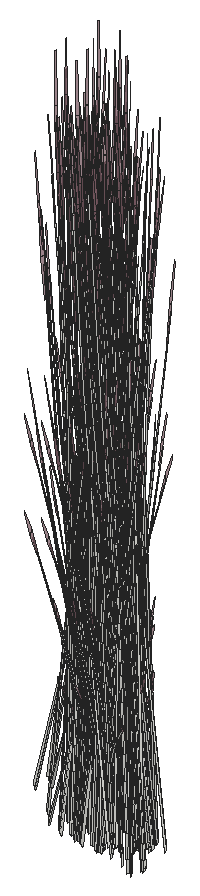
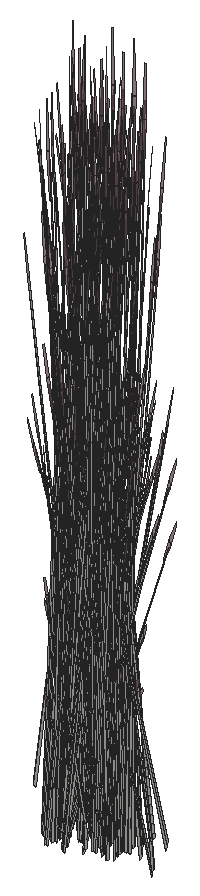
# SketchUp Ruby script. Lengths in inches.
U = 1.inch
M = Sketchup.active_model
def pt(a) = Geom::Point3d.new(a.map { |v| v * U })
def face(e, loops, mat)
  f = e.add_face(loops[0].map { |a| pt(a) })
  loops[1..].each { |l| e.add_face(l.map { |a| pt(a) }).erase! }
  f.material = f.back_material = mat if mat
  f
end
# faces: each face lists its corners as indices into pts; further lists are holes
def faces(e, pts, list, mat = nil) = list.each { |f| face(e, (f[0].is_a?(Array) ? f : [f]).map { |l| l.map { |i| pts[i] } }, mat) }
# xy, xz, yz: faces in a plane at the given z, y or x. An outline is a flat list of corners, or four numbers for a rectangle; further outlines are holes
def ring(l) = l.size == 4 ? [[l[0], l[1]], [l[2], l[1]], [l[2], l[3]], [l[0], l[3]]] : l.each_slice(2).to_a
def flat(e, list, mat, &to3) = list.each { |f| face(e, (f[0].is_a?(Array) ? f : [f]).map { |l| ring(l).map { |u, v| to3.(u, v) } }, mat) }
def xy(e, z, list, mat = nil) = flat(e, list, mat) { |x, y| [x, y, z] }
def xz(e, y, list, mat = nil) = flat(e, list, mat) { |x, z| [x, y, z] }
def yz(e, x, list, mat = nil) = flat(e, list, mat) { |y, z| [x, y, z] }
def lines(e, pts, list) = list.each { |a, b| e.add_line(pt(pts[a]), pt(pts[b])) }
# prism: a flat outline (further loops are holes) pulled along v
def prism(e, loops, v, mat = nil)
  f = face(e, loops, mat); d = Geom::Vector3d.new(v.map { |x| x * U })
  f.pushpull(f.normal.samedirection?(d) ? d.length : -d.length)
end
def box(e, o, s, mat = nil) = prism(e, [[o, [o[0] + s[0], o[1], o[2]], [o[0] + s[0], o[1] + s[1], o[2]], [o[0], o[1] + s[1], o[2]]]], [0, 0, s[2]], mat)
def at(x, y, z, deg = 0) = Geom::Transformation.translation(pt([x, y, z])) * Geom::Transformation.rotation(ORIGIN, Z_AXIS, deg.degrees)
def axes(o, x, y, z) = Geom::Transformation.new([*x, 0, *y, 0, *z, 0, *pt(o).to_a, 1])
def part(name) = M.definitions.add(name)
# library, detail: a bought-in or finely detailed component or shape, given as its bounding box
def library(name, o, s) = part(name).tap { |d| box(d.entities, o, s) }
def detail(e, o, s) = box(e.add_group.entities, o, s)
def put(e, d, t, mat = nil) = e.add_instance(d, t).tap { |i| i.material = mat if mat }
def group(e, t, mat = nil) = e.add_group.tap { |g| g.transformation = t; g.material = mat if mat }.entities
root = M.entities
M.materials.add("LightPink_Translucent").color = [144, 107, 117]
M.materials["LightPink_Translucent"].alpha = 0.75
c1 = part("blade")
p = [[2.15,0.21,22],[0,0.17,0],[0.09,0.45,0],[2.18,0.31,22],[2.29,0.31,22],[0.38,0.45,0],
  [2.48,0.24,33],[2.49,0.24,33],[2.48,0.22,33]]
faces(c1.entities,p,[[0,1,2,3],[4,5,2,3],[6,3,4,7],[8,0,3,6]])
c2 = part("seeds")
p = [[0.3,-0.1,1.38],[-0.01,-0.03,1.59],[-0.01,-0.03,0.03],[0.14,-0.07,-0.07],[0.29,-0.03,3],[0.15,0.01,3.11]]
faces(c2.entities,p,[[0,1,2,3],[1,0,4,5]],"LightPink_Translucent")
c3 = part("blade with seeds")
put(c3.entities,c1,at(0,0,0))
put(c3.entities,c2,axes([2.4,0.25,30.99],[1.5799,-0.05474,1.17369],[-0.12525,1.92788,0.29478],[-0.07173,-0.02425,1.56792]))
put(root,c3,axes([350.7,355.2,622.53],[0.29332,0.1301,-0.35414],[-0.08555,0.37955,0.4572],[0.11809,-0.0348,0.87481]))
put(root,c3,axes([354.22,355.91,620.47],[0.10196,-0.46348,0.17642],[0.3731,0.13116,0.35086],[-0.06445,0.00226,1.60407]))
put(root,c3,axes([353.96,354.95,620.3],[-0.32829,-0.4014,-0.06131],[0.32849,-0.40164,0],[-0.01146,-0.01402,1.75571]))
put(root,c3,axes([356.95,354.6,621.875],[0.14639,-0.01056,1.71376],[-0.09712,0.45778,0.13857],[-0.20862,-0.02831,0.73262]))
put(root,c3,axes([350.85,355.125,619.98],[-0.22732,0.05597,1.41583],[-0.03618,-0.44548,0.08104],[0.15921,-0.06743,0.80566]))
put(root,c3,axes([351.1,354.83,619.49],[-0.01845,-0.0708,1.76342],[0.12793,-0.41416,-0.26939],[0.12905,-0.00596,0.30037]))
put(root,c3,axes([355.63,354.99,620.67],[-0.35635,0.30962,-0.29095],[-0.23697,-0.43749,-0.50002],[-0.08792,-0.04443,1.59708]))
put(root,c3,axes([349.9,354.73,621.875],[-0.14639,0.01056,1.71376],[0.09712,-0.45778,0.13857],[0.20862,0.02831,0.73262]))
put(root,c3,axes([353.3,354.49,620.36],[0.15345,0.52148,0.45755],[-0.43845,0.18134,0.17955],[0.00536,-0.09582,1.58856]))
put(root,c3,axes([353.66,355.78,620.2],[-0.11516,-0.40207,0],[0.32884,-0.1408,0],[0,0,1.54371]))
put(root,c3,axes([354.83,355.64,620.03],[-0.08291,-0.40636,-0.30978],[0.32928,-0.11539,0.30978],[-0.06638,-0.04686,1.38974]))
put(root,c3,axes([350.44,355.16,622.98],[0.31014,-0.20596,-0.71045],[0.17284,0.42397,0.08574],[0.14985,-0.04816,1.00501]))
put(root,c3,axes([351.48,354.71,622.72],[0.04898,-0.07104,1.74944],[-0.06269,-0.43574,-0.27667],[0.12289,-0.08262,0.14031]))
put(root,c3,axes([354.81,354.73,620.47],[-0.2773,-0.3397,0.17642],[0.27945,-0.32949,0.35086],[-0.03063,0.06937,1.60407]))
put(root,c3,axes([356.03,355.13,620.46],[-0.34464,-0.37536,-0.25192],[0.29,-0.42149,0.5513],[-0.0928,0.04391,1.68216]))
put(root,c3,axes([355.41,354.77,620.21],[-0.21202,-0.39143,-0.44739],[0.32115,-0.27564,0.21531],[-0.06861,-0.04843,1.43643]))
put(root,c3,axes([353.85,354.53,620.21],[0,-0.53961,0],[0.44133,0,0],[0,0,1.79456]))
put(root,c3,axes([353.4375,354.63,620.43],[0.39767,0.22603,0.24065],[-0.19139,0.46966,0.50002],[0,-0.10827,1.60543]))
put(root,c3,axes([354.07,354.75,620.29],[0,0.53934,-0.05637],[-0.44133,0,0],[0,0.01695,1.79368]))
put(root,c3,axes([353.31,354.32,620.72],[-0.38326,0.02879,0.44739],[-0.03466,-0.47788,-0.21531],[0.06861,-0.04843,1.43643]))
put(root,c3,axes([355.86,355.05,620.21],[-0.38326,0.02879,-0.44739],[-0.03466,-0.47788,0.21531],[-0.06861,0.04843,1.43643]))
put(root,c3,axes([353.13,353.5,620.47],[-0.10196,0.46348,0.17642],[-0.3731,-0.13116,0.35086],[0.06445,-0.00226,1.60407]))
put(root,c3,axes([357.39,354.17,622.98],[-0.35281,-0.01123,-0.71045],[0.0237,-0.47284,0.08574],[-0.14947,-0.0499,1.00501]))
put(root,c3,axes([355.13,355.85,620.48],[0.33032,0.23318,0.49651],[-0.19744,0.41812,0],[-0.07523,-0.05311,1.57504]))
put(root,c3,axes([357.1,354.28,620.59],[0.06891,0.12984,1.43002],[-0.15879,0.35293,-0.30754],[-0.16304,-0.08436,0.61141]))
put(root,c3,axes([355.4375,354.99,620.4375],[0.09355,-0.55261,-0.23429],[0.44354,0.09633,0.51271],[-0.0775,-0.07631,1.5644]))
put(root,c3,axes([356.82,354.99,622.53],[-0.29332,-0.1301,-0.35414],[0.08555,-0.37955,0.4572],[-0.11809,0.0348,0.87481]))
put(root,c3,axes([354.26,353.52,620.47],[-0.37926,0.12378,0.17642],[-0.09365,-0.46065,0.35086],[0.03382,0.06712,1.60407]))
put(root,c3,axes([355.6,355.125,620.62],[-0.06809,0.4162,0.1448],[-0.33266,-0.07225,-0.41347],[-0.06054,-0.04274,1.26744]))
put(root,c3,axes([354.48,354.39,620.48],[0,0.46636,0.49651],[-0.39487,0,0],[0,-0.10622,1.57504]))
put(root,c3,axes([353.64,354.19,620.36],[-0.29264,0.42323,0.45755],[-0.34767,-0.3736,0.17955],[0.07055,-0.04224,1.58856]))
put(root,c3,axes([354.14,354.86,620.21],[0.24637,0.30123,0],[-0.24637,0.30123,0],[0,0,1.69266]))
put(root,c3,axes([354.13,354.51,620.72],[0.17124,-0.42022,0.44739],[0.35581,0.20224,-0.21531],[0,0.09687,1.43643]))
put(root,c3,axes([357.27,354.27,622.68],[-0.25628,0.30892,-0.51099],[-0.22444,-0.32634,-0.3958],[-0.13021,-0.047,0.97773]))
put(root,c3,axes([356.86,355.16,619.49],[0.00895,0.0735,1.76342],[-0.18044,0.38382,-0.26939],[-0.12817,-0.01935,0.30037]))
put(root,c3,axes([354.02,354.41,620.38],[-0.44609,-0.09826,0.49198],[0.09078,-0.55493,0.19306],[0.06519,0.05359,1.70813]))
put(root,c3,axes([356.91,353.4,622.71],[0.02617,0.04654,1.77383],[-0.12614,0.41836,-0.16761],[-0.12775,0.00303,0.31391]))
put(root,c3,axes([354.15,354.66,620.21],[0.39487,0,0],[0,0.48281,0],[0,0,1.78407]))
put(root,c3,axes([356.89,354.94,622.73],[0.09971,-0.42522,0.48003],[0.32782,0.1454,0.3958],[-0.12892,0.02555,0.9933]))
put(root,c3,axes([353.77,354.12,620.72],[-0.21202,-0.39143,0.44739],[0.32115,-0.27564,-0.21531],[0.06861,0.04843,1.43643]))
put(root,c3,axes([357.41,353.94,623.03],[-0.0189,0.47427,-0.1216],[-0.35781,-0.01296,-0.67495],[-0.13781,-0.03295,1.02557]))
put(root,c3,axes([357.18,353.97,622.53],[-0.20082,-0.29199,-0.35414],[0.2293,-0.2764,0.4572],[-0.1165,-0.04206,0.87481]))
put(root,c3,axes([356.86,354.83,622.73],[-0.12963,-0.31798,0.0643],[0.23638,-0.15564,0.50621],[-0.1042,0.03071,0.77189]))
put(root,c3,axes([358.49,354.61,621.875],[0.14639,-0.01056,1.71376],[-0.09712,0.45778,0.13857],[-0.20862,-0.02831,0.73262]))
put(root,c3,axes([355.49,354.73,620.36],[0.44609,0.09826,0.45755],[-0.09078,0.55493,0.17955],[-0.06519,-0.05359,1.58856]))
put(root,c3,axes([356.69,354.67,620.77],[0.22533,-0.03337,1.1486],[-0.14293,0.29403,0.84392],[-0.11135,-0.04411,0.25299]))
put(root,c3,axes([355.375,354.63,620.72],[-0.17124,0.42022,0.44739],[-0.35581,-0.20224,-0.21531],[0,-0.09687,1.43643]))
put(root,c3,axes([353.91,354.01,620.62],[0.06809,-0.4162,0.1448],[0.33266,0.07225,-0.41347],[0.06054,0.04274,1.26744]))
put(root,c3,axes([355.25,355.61,620.47],[0.37926,-0.12378,0.17642],[0.09365,0.46065,0.35086],[-0.03382,-0.06712,1.60407]))
put(root,c3,axes([355.74,355.6875,620.2],[-0.35581,-0.20937,0],[0.17124,-0.43505,0],[0,0,1.62707]))
put(root,c3,axes([354.38,353.29,620.48],[-0.33032,-0.23318,0.49651],[0.19744,-0.41812,0],[0.07523,0.05311,1.57504]))
put(root,c3,axes([354.09,355.72,620.18],[0.37054,-0.15823,-0.19198],[0.1302,0.45581,0.00008],[0.0409,-0.01749,1.73897]))
put(root,c3,axes([357.13,354.95,623.05],[0.29332,0.1301,0.35414],[-0.08555,0.37955,-0.4572],[-0.11809,0.0348,0.87481]))
put(root,c3,axes([356.38,355.64,620.47],[0.10196,-0.46348,0.17642],[0.3731,0.13116,0.35086],[-0.06445,0.00226,1.60407]))
put(root,c3,axes([357.28,353.86,622.73],[0.01777,-0.35463,0.0643],[0.26836,0.00972,0.50621],[-0.1028,-0.03711,0.77189]))
put(root,c3,axes([356.11,354.68,620.3],[-0.32829,-0.4014,-0.06131],[0.32849,-0.40164,0],[-0.01146,-0.01402,1.75571]))
put(root,c3,axes([356.2,354.82,620.72],[0.38326,-0.02879,0.44739],[0.03466,0.47788,-0.21531],[-0.06861,0.04843,1.43643]))
put(root,c3,axes([358.04,355.82,620.06],[-0.36714,-0.07646,-0.62353],[0.07747,-0.47163,-0.16365],[-0.10956,-0.05715,1.37633]))
put(root,c3,axes([354.1,354.37,620.21],[0.21202,0.39143,-0.44739],[-0.32115,0.27564,0.21531],[0.06861,0.04843,1.43643]))
put(root,c3,axes([357.46,354.13,623.05],[0.20082,0.29199,0.35414],[-0.2293,0.2764,-0.4572],[-0.1165,-0.04206,0.87481]))
put(root,c3,axes([355.45,354.22,620.36],[0.15345,0.52148,0.45755],[-0.43845,0.18134,0.17955],[0.00536,-0.09582,1.58856]))
put(root,c3,axes([358.92,354.18,622.98],[-0.35281,-0.01123,-0.71045],[0.0237,-0.47284,0.08574],[-0.14947,-0.0499,1.00501]))
put(root,c3,axes([355.82,355.51,620.2],[-0.11516,-0.40207,0],[0.32884,-0.1408,0],[0,0,1.54371]))
put(root,c3,axes([358.64,354.3,620.59],[0.06891,0.12984,1.43002],[-0.15879,0.35293,-0.30754],[-0.16304,-0.08436,0.61141]))
put(root,c3,axes([357.56,356.71,620.02],[-0.33032,-0.23318,-0.49651],[0.19744,-0.41812,0],[-0.07523,-0.05311,1.57504]))
put(root,c3,axes([359.07,351.34,621.875],[0.12246,-0.09864,1.71376],[0.1031,0.45582,0.13857],[-0.19225,0.10302,0.73262]))
put(root,c3,axes([358.36,355,622.53],[-0.29332,-0.1301,-0.35414],[0.08555,-0.37955,0.4572],[-0.11809,0.0348,0.87481]))
put(root,c3,axes([358.6875,352.12,620.59],[0.12266,0.03828,1.43002],[0.07906,0.39104,-0.30754],[-0.16661,0.0732,0.61141]))
put(root,c3,axes([354.68,353.5,620.03],[0.08291,0.40636,-0.30978],[-0.32928,0.11539,0.30978],[0.06638,0.04686,1.38974]))
put(root,c3,axes([353.875,354.15,620.67],[0.35635,-0.30962,-0.29095],[0.23697,0.43749,-0.50002],[0.08792,0.04443,1.59708]))
put(root,c3,axes([358.81,354.28,622.68],[-0.25628,0.30892,-0.51099],[-0.22444,-0.32634,-0.3958],[-0.13021,-0.047,0.97773]))
put(root,c3,axes([358.39,355.17,619.49],[0.00895,0.0735,1.76342],[-0.18044,0.38382,-0.26939],[-0.12817,-0.01935,0.30037]))
put(root,c3,axes([356.96,354.46,620.47],[-0.2773,-0.3397,0.17642],[0.27945,-0.32949,0.35086],[-0.03063,0.06937,1.60407]))
put(root,c3,axes([356,354.26,620.21],[0,-0.53961,0],[0.44133,0,0],[0,0,1.79456]))
put(root,c3,axes([357.2,353.48,620.13],[-0.10181,0.3808,-0.03893],[-0.31336,-0.11714,-0.17649],[-0.04758,-0.06228,0.58215]))
put(root,c3,axes([355.59,354.36,620.43],[0.39767,0.22603,0.24065],[-0.19139,0.46966,0.50002],[0,-0.10827,1.60543]))
put(root,c3,axes([356.23,354.48,620.29],[0,0.53934,-0.05637],[-0.44133,0,0],[0,0.01695,1.79368]))
put(root,c3,axes([358.44,353.41,622.71],[0.02617,0.04654,1.77383],[-0.12614,0.41836,-0.16761],[-0.12775,0.00303,0.31391]))
put(root,c3,axes([355.47,354.04,620.72],[-0.38326,0.02879,0.44739],[-0.03466,-0.47788,-0.21531],[0.06861,-0.04843,1.43643]))
put(root,c3,axes([355.29,353.22,620.47],[-0.10196,0.46348,0.17642],[-0.3731,-0.13116,0.35086],[0.06445,-0.00226,1.60407]))
put(root,c3,axes([358.45,355.89,620.67],[-0.35635,0.30962,-0.29095],[-0.23697,-0.43749,-0.50002],[-0.08792,-0.04443,1.59708]))
put(root,c3,axes([358.43,354.95,622.73],[0.09971,-0.42522,0.48003],[0.32782,0.1454,0.3958],[-0.12892,0.02555,0.9933]))
put(root,c3,axes([352.98,353.87,619.59],[-0.3474,0.18671,1.28929],[-0.11057,-0.53572,0.50096],[0.21332,0.00891,1.46642]))
put(root,c3,axes([358.94,353.95,623.03],[-0.0189,0.47427,-0.1216],[-0.35781,-0.01296,-0.67495],[-0.13781,-0.03295,1.02557]))
put(root,c3,axes([358.71,353.99,622.53],[-0.20082,-0.29199,-0.35414],[0.2293,-0.2764,0.4572],[-0.1165,-0.04206,0.87481]))
put(root,c3,axes([358.4,354.84,622.73],[-0.12963,-0.31798,0.0643],[0.23638,-0.15564,0.50621],[-0.1042,0.03071,0.77189]))
put(root,c3,axes([357.03,355.22,620.375],[-0.44133,0,0],[0,-0.52122,-0.51607],[0,-0.11871,1.63711]))
put(root,c3,axes([357.65,356.54,620.03],[-0.08291,-0.40636,-0.30978],[0.32928,-0.11539,0.30978],[-0.06638,-0.04686,1.38974]))
put(root,c3,axes([356.42,353.25,620.47],[-0.37926,0.12378,0.17642],[-0.09365,-0.46065,0.35086],[0.03382,0.06712,1.60407]))
put(root,c3,axes([358.05,351.63,622.71],[0.04504,0.01251,1.77383],[0.13934,0.41205,-0.16761],[-0.0922,0.10815,0.31391]))
put(root,c3,axes([354.57,353.04,620.375],[0.22066,-0.46731,0],[0.36918,0.26061,-0.51607],[0.08408,0.05936,1.63711]))
put(root,c3,axes([358.23,354.6875,620.77],[0.22533,-0.03337,1.1486],[-0.14293,0.29403,0.84392],[-0.11135,-0.04411,0.25299]))
put(root,c3,axes([354.77,353.32,620.02],[0.33032,0.23318,-0.49651],[-0.19744,0.41812,0],[0.07523,0.05311,1.57504]))
put(root,c3,axes([355.79,353.92,620.36],[-0.29264,0.42323,0.45755],[-0.34767,-0.3736,0.17955],[0.07055,-0.04224,1.58856]))
put(root,c3,axes([356.29,354.59,620.21],[0.24637,0.30123,0],[-0.24637,0.30123,0],[0,0,1.69266]))
put(root,c3,axes([356.29,354.24,620.72],[0.17124,-0.42022,0.44739],[0.35581,0.20224,-0.21531],[0,0.09687,1.43643]))
put(root,c3,axes([357.37,355.08,620.33],[-0.32829,0.39208,0.30756],[-0.32849,-0.38796,-0.36492],[-0.01146,-0.11134,1.64885]))
put(root,c3,axes([355.54,356.02,621.93],[-0.06755,-0.39203,-0.03492],[0.31928,-0.09013,-0.15832],[0.06667,0.02485,0.52218]))
put(root,c3,axes([354.98,355.01,623.05],[-0.29332,-0.1301,0.35414],[0.08555,-0.37955,-0.4572],[0.11809,-0.0348,0.87481]))
put(root,c3,axes([358.43,352.94,620.77],[0.14709,-0.21136,1.1486],[0.05804,0.3346,0.84392],[-0.1063,0.05991,0.25299]))
put(root,c3,axes([356.18,354.14,620.38],[-0.44609,-0.09826,0.49198],[0.09078,-0.55493,0.19306],[0.06519,0.05359,1.70813]))
put(root,c3,axes([358.23,355.67,620.21],[-0.21202,-0.39143,-0.44739],[0.32115,-0.27564,0.21531],[-0.06861,-0.04843,1.43643]))
put(root,c3,axes([354.29,354.22,620.06],[0.36714,0.07646,-0.62353],[-0.07747,0.47163,-0.16365],[0.10956,0.05715,1.37633]))
put(root,c3,axes([355.86,354.5,620.26],[-0.21881,-0.29821,-0.06488],[0.23965,-0.27324,-0.29416],[0.0679,-0.01924,0.97024]))
put(root,c3,axes([356.3,354.38,620.21],[0.39487,0,0],[0,0.48281,0],[0,0,1.78407]))
put(root,c3,axes([359.52,351.65,621.875],[0.08815,-0.14329,1.71376],[0.22258,0.38678,0.13857],[-0.15267,0.17614,0.73262]))
put(root,c3,axes([355.92,353.85,620.72],[-0.21202,-0.39143,0.44739],[0.32115,-0.27564,-0.21531],[0.06861,0.04843,1.43643]))
put(root,c3,axes([358.99,352.03,622.53],[-0.30722,0.06665,-0.35414],[-0.08112,-0.381,0.4572],[-0.08804,0.10234,0.87481]))
put(root,c3,axes([358.67,354.96,623.05],[0.29332,0.1301,0.35414],[-0.08555,0.37955,-0.4572],[-0.11809,0.0348,0.87481]))
put(root,c3,axes([356.44,354.33,620.62],[0.32884,-0.136,0.1448],[0.11516,0.38837,-0.41347],[0,0.08547,1.26744]))
put(root,c3,axes([355.21,354.03,622.73],[0.2423,0.19613,0.0643],[-0.14107,0.2793,0.50621],[0.07768,-0.0903,0.77189]))
put(root,c3,axes([358.82,353.16,619.49],[0.04734,0.04659,1.76342],[0.08027,0.4317,-0.26939],[-0.10492,0.09206,0.30037]))
put(root,c3,axes([355.15,353.95,622.73],[0.08753,0.42921,0.48003],[-0.34336,0.07449,0.3958],[0.1012,-0.10094,0.9933]))
put(root,c3,axes([358.8125,353.875,622.73],[0.01777,-0.35463,0.0643],[0.26836,0.00972,0.50621],[-0.1028,-0.03711,0.77189]))
put(root,c3,axes([359.57,355.83,620.06],[-0.36714,-0.07646,-0.62353],[0.07747,-0.47163,-0.16365],[-0.10956,-0.05715,1.37633]))
put(root,c3,axes([358.26,355.9,620.4375],[0.09355,-0.55261,-0.23429],[0.44354,0.09633,0.51271],[-0.0775,-0.07631,1.5644]))
put(root,c3,axes([359,354.14,623.05],[0.20082,0.29199,0.35414],[-0.2293,0.2764,-0.4572],[-0.1165,-0.04206,0.87481]))
put(root,c3,axes([359.03,351.94,622.73],[-0.08753,-0.42921,0.48003],[0.34336,-0.07449,0.3958],[-0.1012,0.10094,0.9933]))
put(root,c3,axes([358.42,356.03,620.62],[-0.06809,0.4162,0.1448],[-0.33266,-0.07225,-0.41347],[-0.06054,-0.04274,1.26744]))
put(root,c3,axes([357.3,355.3,620.48],[0,0.46636,0.49651],[-0.39487,0,0],[0,-0.10622,1.57504]))
put(root,c3,axes([358.96,351.86,622.73],[-0.2423,-0.19613,0.0643],[0.14107,-0.2793,0.50621],[-0.07768,0.0903,0.77189]))
put(root,c3,axes([357.19,354.47,620.48],[0,-0.46636,0.49651],[0.39487,0,0],[0,0.10622,1.57504]))
put(root,c3,axes([355.25,355.125,622.73],[0.12963,0.31798,0.0643],[-0.23638,0.15564,0.50621],[0.1042,-0.03071,0.77189]))
put(root,c3,axes([359.09,356.73,620.02],[-0.33032,-0.23318,-0.49651],[0.19744,-0.41812,0],[-0.07523,-0.05311,1.57504]))
put(root,c3,axes([354.71,356.01,623.03],[0.0189,-0.47427,-0.1216],[0.35781,0.01296,-0.67495],[0.13781,0.03295,1.02557]))
put(root,c3,axes([355.11,355.13,623.03],[-0.17758,-0.42229,-0.1216],[0.31518,-0.20752,-0.67495],[0.13282,-0.05572,1.02557]))
put(root,c3,axes([356.07,353.74,620.62],[0.06809,-0.4162,0.1448],[0.33266,0.07225,-0.41347],[0.06054,0.04274,1.26744]))
put(root,c3,axes([355.22,355.01,622.73],[-0.09971,0.42522,0.48003],[-0.32782,-0.1454,0.3958],[0.12892,-0.02555,0.9933]))
put(root,c3,axes([359.45,352.01,621.875],[0.06572,-0.16029,1.71376],[0.27569,0.33172,0.13857],[-0.12437,0.20675,0.73262]))
put(root,c3,axes([358.16,355.4,620.67],[-0.39748,-0.22252,-0.29095],[0.19139,-0.46966,-0.50002],[-0.01249,-0.11531,1.59708]))
put(root,c3,axes([356.54,353.01,620.48],[-0.33032,-0.23318,0.49651],[0.19744,-0.41812,0],[0.07523,0.05311,1.57504]))
put(root,c3,axes([359.24,352.07,622.68],[0.09067,0.42583,-0.51099],[-0.34336,0.07449,-0.3958],[-0.0984,0.11438,0.97773]))
put(root,c3,axes([356.25,355.45,620.18],[0.37054,-0.15823,-0.19198],[0.1302,0.45581,0.00008],[0.0409,-0.01749,1.73897]))
put(root,c3,axes([358.7,352.84,622.72],[-0.00877,0.09229,1.74944],[0.24897,0.32105,-0.27667],[-0.06518,0.15182,0.14031]))
put(root,c3,axes([358.73,353.49,620.13],[-0.10181,0.3808,-0.03893],[-0.31336,-0.11714,-0.17649],[-0.04758,-0.06228,0.58215]))
put(root,c3,axes([355.09,354.77,622.68],[0.09562,-0.42421,-0.51099],[0.32782,0.1454,-0.3958],[0.13199,-0.0389,0.97773]))
put(root,c3,axes([357.3,354.87,620.03],[0.24637,-0.29097,-0.30978],[0.24637,0.29097,0.30978],[0,-0.09372,1.38974]))
put(root,c3,axes([355.91,355.04,620.77],[-0.21807,0.07699,1.1486],[0.10265,-0.31819,0.84392],[0.11568,0.02177,0.25299]))
put(root,c3,axes([356.26,354.09,620.21],[0.21202,0.39143,-0.44739],[-0.32115,0.27564,0.21531],[0.06861,0.04843,1.43643]))
put(root,c3,axes([358.31,355.63,620.36],[0.44609,0.09826,0.45755],[-0.09078,0.55493,0.17955],[-0.06519,-0.05359,1.58856]))
put(root,c3,axes([359.99,355.9,620.67],[-0.35635,0.30962,-0.29095],[-0.23697,-0.43749,-0.50002],[-0.08792,-0.04443,1.59708]))
put(root,c3,axes([355.29,354.96,622.53],[0.29332,0.1301,-0.35414],[-0.08555,0.37955,0.4572],[0.11809,-0.0348,0.87481]))
put(root,c3,axes([359.08,351.77,623.03],[0.32648,0.25715,-0.1216],[-0.18809,0.3724,-0.67495],[-0.09224,0.12945,1.02557]))
put(root,c3,axes([358.19,355.53,620.72],[-0.17124,0.42022,0.44739],[-0.35581,-0.20224,-0.21531],[0,-0.09687,1.43643]))
put(root,c3,axes([358.5625,355.23,620.375],[-0.44133,0,0],[0,-0.52122,-0.51607],[0,-0.11871,1.63711]))
put(root,c3,axes([359.18,356.55,620.03],[-0.08291,-0.40636,-0.30978],[0.32928,-0.11539,0.30978],[-0.06638,-0.04686,1.38974]))
put(root,c3,axes([355.44,354.89,619.98],[-0.22732,0.05597,1.41583],[-0.03618,-0.44548,0.08104],[0.15921,-0.06743,0.80566]))
put(root,c3,axes([358.07,356.52,620.47],[0.37926,-0.12378,0.17642],[0.09365,0.46065,0.35086],[-0.03382,-0.06712,1.60407]))
put(root,c3,axes([355.6875,354.6,619.49],[-0.01845,-0.0708,1.76342],[0.12793,-0.41416,-0.26939],[0.12905,-0.00596,0.30037]))
put(root,c3,axes([358.54,352.88,623.65],[0.31145,0.12449,-0.06488],[-0.0958,0.38314,-0.29416],[-0.05094,0.05817,0.97024]))
put(root,c3,axes([355.8125,356.39,622.71],[-0.03191,-0.04083,1.77383],[0.06981,-0.43764,-0.16761],[0.12571,-0.02796,0.31391]))
put(root,c3,axes([354.49,354.49,621.875],[-0.14639,0.01056,1.71376],[0.09712,-0.45778,0.13857],[0.20862,0.02831,0.73262]))
put(root,c3,axes([356.84,353.23,620.03],[0.08291,0.40636,-0.30978],[-0.32928,0.11539,0.30978],[0.06638,0.04686,1.38974]))
put(root,c3,axes([359.24,351.8,623.05],[0.30722,-0.06665,0.35414],[0.08112,0.381,-0.4572],[-0.08804,0.10234,0.87481]))
put(root,c3,axes([358.91,355.09,620.33],[-0.32829,0.39208,0.30756],[-0.32849,-0.38796,-0.36492],[-0.01146,-0.11134,1.64885]))
put(root,c3,axes([356.03,353.875,620.67],[0.35635,-0.30962,-0.29095],[0.23697,0.43749,-0.50002],[0.08792,0.04443,1.59708]))
put(root,c3,axes([355.03,354.93,622.98],[0.31014,-0.20596,-0.71045],[0.17284,0.42397,0.08574],[0.14985,-0.04816,1.00501]))
put(root,c3,axes([359.2,356.54,620.47],[0.10196,-0.46348,0.17642],[0.3731,0.13116,0.35086],[-0.06445,0.00226,1.60407]))
put(root,c3,axes([359.76,355.68,620.21],[-0.21202,-0.39143,-0.44739],[0.32115,-0.27564,0.21531],[-0.06861,-0.04843,1.43643]))
put(root,c3,axes([358.93,355.58,620.3],[-0.32829,-0.4014,-0.06131],[0.32849,-0.40164,0],[-0.01146,-0.01402,1.75571]))
put(root,c3,axes([356.07,354.47,622.72],[0.04898,-0.07104,1.74944],[-0.06269,-0.43574,-0.27667],[0.12289,-0.08262,0.14031]))
put(root,c3,axes([359.53,352.8125,622.73],[-0.25132,-0.3182,0.48003],[0.2669,-0.27442,0.3958],[-0.04636,0.14929,0.9933]))
put(root,c3,axes([359.43,352.78,622.73],[-0.29004,-0.02173,0.0643],[0.00795,-0.32812,0.50621],[-0.03035,0.12569,0.77189]))
put(root,c3,axes([355.13,353.6,619.59],[-0.3474,0.18671,1.28929],[-0.11057,-0.53572,0.50096],[0.21332,0.00891,1.46642]))
put(root,c3,axes([358.27,355.12,620.36],[0.15345,0.52148,0.45755],[-0.43845,0.18134,0.17955],[0.00536,-0.09582,1.58856]))
put(root,c3,axes([359.53,352.91,622.53],[-0.23881,0.24554,-0.35414],[-0.22606,-0.28036,0.4572],[-0.0344,0.14245,0.87481]))
put(root,c3,axes([358.2,355.05,620.21],[0.17124,-0.42022,-0.44739],[0.35581,0.20224,0.21531],[0,-0.09687,1.43643]))
put(root,c3,axes([358.64,356.41,620.2],[-0.11516,-0.40207,0],[0.32884,-0.1408,0],[0,0,1.54371]))
put(root,c3,axes([359.8,355.91,620.4375],[0.09355,-0.55261,-0.23429],[0.44354,0.09633,0.51271],[-0.0775,-0.07631,1.5644]))
put(root,c3,axes([360.75,352.17,620.06],[-0.23773,0.35053,-0.62353],[-0.29532,-0.31785,-0.16365],[-0.09526,0.08744,1.37633]))
put(root,c3,axes([356.73,352.77,620.375],[0.22066,-0.46731,0],[0.36918,0.26061,-0.51607],[0.08408,0.05936,1.63711]))
put(root,c3,axes([356.81,355.55,623.05],[-0.20082,-0.29199,0.35414],[0.2293,-0.2764,-0.4572],[0.1165,0.04206,0.87481]))
put(root,c3,axes([359.96,356.04,620.62],[-0.06809,0.4162,0.1448],[-0.33266,-0.07225,-0.41347],[-0.06054,-0.04274,1.26744]))
put(root,c3,axes([356.93,353.05,620.02],[0.33032,0.23318,-0.49651],[-0.19744,0.41812,0],[0.07523,0.05311,1.57504]))
put(root,c3,axes([358.83,355.31,620.48],[0,0.46636,0.49651],[-0.39487,0,0],[0,-0.10622,1.57504]))
put(root,c3,axes([357.69,355.75,621.93],[-0.06755,-0.39203,-0.03492],[0.31928,-0.09013,-0.15832],[0.06667,0.02485,0.52218]))
put(root,c3,axes([357.14,354.73,623.05],[-0.29332,-0.1301,0.35414],[0.08555,-0.37955,-0.4572],[0.11809,-0.0348,0.87481]))
put(root,c3,axes([359.68,353.86,620.77],[-0.00913,-0.2773,1.1486],[0.22824,0.19778,0.84392],[-0.04489,0.13217,0.25299]))
put(root,c3,axes([358.82,355.16,620.21],[0,-0.53961,0],[0.44133,0,0],[0,0,1.79456]))
put(root,c3,axes([359.69,355.41,620.67],[-0.39748,-0.22252,-0.29095],[0.19139,-0.46966,-0.50002],[-0.01249,-0.11531,1.59708]))
put(root,c3,axes([360.74,351.9,620.21],[-0.38326,0.02879,-0.44739],[-0.03466,-0.47788,0.21531],[-0.06861,0.04843,1.43643]))
put(root,c3,axes([356.45,353.94,620.06],[0.36714,0.07646,-0.62353],[-0.07747,0.47163,-0.16365],[0.10956,0.05715,1.37633]))
put(root,c3,axes([358.41,355.26,620.43],[0.39767,0.22603,0.24065],[-0.19139,0.46966,0.50002],[0,-0.10827,1.60543]))
put(root,c3,axes([358.29,354.95,620.72],[-0.38326,0.02879,0.44739],[-0.03466,-0.47788,-0.21531],[0.06861,-0.04843,1.43643]))
put(root,c3,axes([358.01,354.22,620.26],[-0.21881,-0.29821,-0.06488],[0.23965,-0.27324,-0.29416],[0.0679,-0.01924,0.97024]))
put(root,c3,axes([358.11,354.125,620.47],[-0.10196,0.46348,0.17642],[-0.3731,-0.13116,0.35086],[0.06445,-0.00226,1.60407]))
put(root,c3,axes([358.83,354.89,620.03],[0.24637,-0.29097,-0.30978],[0.24637,0.29097,0.30978],[0,-0.09372,1.38974]))
put(root,c3,axes([361.14,353.13,620.02],[-0.33032,0.23318,-0.49651],[-0.19744,-0.41812,0],[-0.07523,0.05311,1.57504]))
put(root,c3,axes([361.16,353.01,620.19],[-0.21791,-0.46895,-0.05142],[0.36918,-0.26061,0.51607],[-0.09097,0.04465,1.6363]))
put(root,c3,axes([359.24,354.15,620.47],[-0.37926,0.12378,0.17642],[-0.09365,-0.46065,0.35086],[0.03382,0.06712,1.60407]))
put(root,c3,axes([359.85,355.64,620.36],[0.44609,0.09826,0.45755],[-0.09078,0.55493,0.17955],[-0.06519,-0.05359,1.58856]))
put(root,c3,axes([358.61,354.82,620.36],[-0.29264,0.42323,0.45755],[-0.34767,-0.3736,0.17955],[0.07055,-0.04224,1.58856]))
put(root,c3,axes([362.68,353.2,621.875],[0.12246,-0.09864,1.71376],[0.1031,0.45582,0.13857],[-0.19225,0.10302,0.73262]))
put(root,c3,axes([361.0625,352.95,620.03],[-0.32928,-0.11539,-0.30978],[0.08291,-0.40636,0.30978],[-0.06638,0.04686,1.38974]))
put(root,c3,axes([359.73,355.54,620.72],[-0.17124,0.42022,0.44739],[-0.35581,-0.20224,-0.21531],[0,-0.09687,1.43643]))
